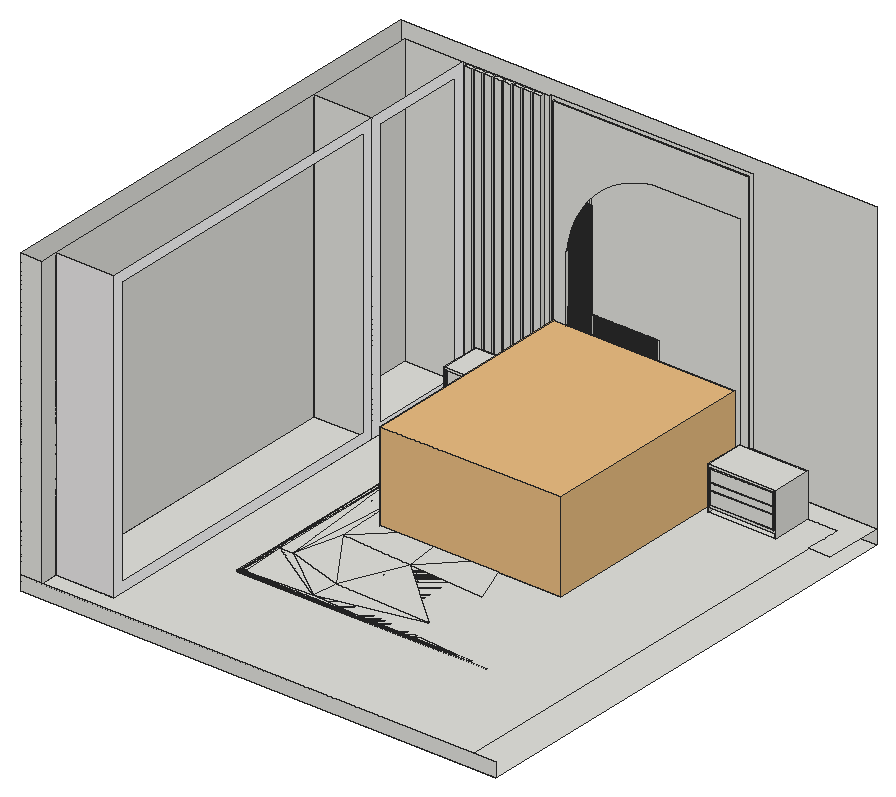
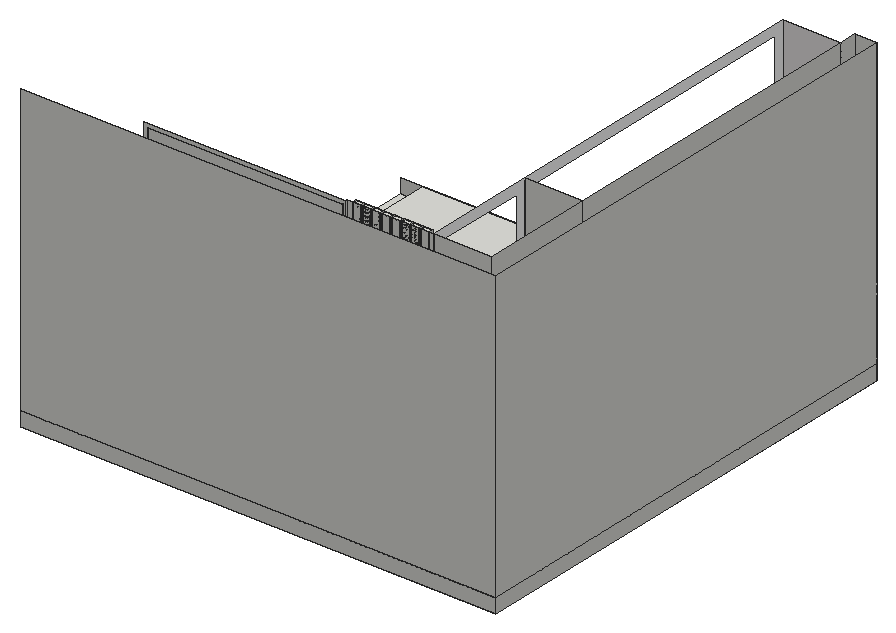
# SketchUp Ruby script. Lengths in inches.
U = 1.inch
M = Sketchup.active_model
def pt(a) = Geom::Point3d.new(a.map { |v| v * U })
def face(e, loops, mat)
  f = e.add_face(loops[0].map { |a| pt(a) })
  loops[1..].each { |l| e.add_face(l.map { |a| pt(a) }).erase! }
  f.material = f.back_material = mat if mat
  f
end
# faces: each face lists its corners as indices into pts; further lists are holes
def faces(e, pts, list, mat = nil) = list.each { |f| face(e, (f[0].is_a?(Array) ? f : [f]).map { |l| l.map { |i| pts[i] } }, mat) }
# xy, xz, yz: faces in a plane at the given z, y or x. An outline is a flat list of corners, or four numbers for a rectangle; further outlines are holes
def ring(l) = l.size == 4 ? [[l[0], l[1]], [l[2], l[1]], [l[2], l[3]], [l[0], l[3]]] : l.each_slice(2).to_a
def flat(e, list, mat, &to3) = list.each { |f| face(e, (f[0].is_a?(Array) ? f : [f]).map { |l| ring(l).map { |u, v| to3.(u, v) } }, mat) }
def xy(e, z, list, mat = nil) = flat(e, list, mat) { |x, y| [x, y, z] }
def xz(e, y, list, mat = nil) = flat(e, list, mat) { |x, z| [x, y, z] }
def yz(e, x, list, mat = nil) = flat(e, list, mat) { |y, z| [x, y, z] }
def lines(e, pts, list) = list.each { |a, b| e.add_line(pt(pts[a]), pt(pts[b])) }
# prism: a flat outline (further loops are holes) pulled along v
def prism(e, loops, v, mat = nil)
  f = face(e, loops, mat); d = Geom::Vector3d.new(v.map { |x| x * U })
  f.pushpull(f.normal.samedirection?(d) ? d.length : -d.length)
end
def box(e, o, s, mat = nil) = prism(e, [[o, [o[0] + s[0], o[1], o[2]], [o[0] + s[0], o[1] + s[1], o[2]], [o[0], o[1] + s[1], o[2]]]], [0, 0, s[2]], mat)
def at(x, y, z, deg = 0) = Geom::Transformation.translation(pt([x, y, z])) * Geom::Transformation.rotation(ORIGIN, Z_AXIS, deg.degrees)
def axes(o, x, y, z) = Geom::Transformation.new([*x, 0, *y, 0, *z, 0, *pt(o).to_a, 1])
def part(name) = M.definitions.add(name)
# library, detail: a bought-in or finely detailed component or shape, given as its bounding box
def library(name, o, s) = part(name).tap { |d| box(d.entities, o, s) }
def detail(e, o, s) = box(e.add_group.entities, o, s)
def put(e, d, t, mat = nil) = e.add_instance(d, t).tap { |i| i.material = mat if mat }
def group(e, t, mat = nil) = e.add_group.tap { |g| g.transformation = t; g.material = mat if mat }.entities
root = M.entities
M.materials.add("Generic").color = [234, 232, 232]
M.materials.add("[Color M00]").color = [255, 255, 255]
c1 = library("Bed 001",[-37.84,-46.07,0],[75.19,90.39,37.01])
xy(root,-6,[[0,0,198,198]])
xy(root,0,[[0,0,9,0,9,189,69.06,189,69.06,189.875,153.17,189.875,153.17,189,171.08,189,171.08,190.5,173.42,190.5,173.42,189,189,189,189,174,198,174,198,198,0,198],[9,0,189,0,189,189,176.63,189,176.63,172.375,148.19,172.375,148.19,189,153.17,189,153.17,189.875,69.06,189.875,69.06,189,33,189,33,7.36,9,7.36],[9,7.36,33,141.67],[54.68,45.79,53.76,45.82,54.37,46.18],[54.68,45.79,54.37,46.18,54.98,46.18],
  [54.68,45.79,54.98,46.18,71.8,46.18],[54.68,45.79,71.8,46.18,79.4375,45.79],[79.4375,45.79,71.8,46.18,129.55,46.18],[53.76,45.82,53.42,45.84,53.76,46.18],[53.76,45.82,53.76,46.18,54.37,46.18],
  [53.42,45.84,53.4,46.18,53.76,46.18],[53.4,46.18,53.37,47.09,53.76,46.79],[53.4,46.18,53.76,46.79,53.76,46.18],[53.76,46.18,53.76,46.79,54.37,46.18],[54.37,46.18,53.76,46.79,54.37,46.79],
  [54.37,46.18,54.37,46.79,54.98,46.18],[54.98,46.18,54.37,46.79,54.98,46.79],[54.98,46.18,54.98,46.79,70.45,46.79],[54.98,46.18,70.45,46.79,71.8,46.18],[71.8,46.18,70.45,46.79,142.125,46.79],
  [53.76,46.79,53.37,47.09,53.76,47.4],[53.76,46.79,53.76,47.4,54.37,46.79],[54.37,46.79,53.76,47.4,54.37,47.4],[54.37,46.79,54.37,47.4,54.98,46.79],[54.98,46.79,54.37,47.4,54.98,47.97],
  [54.98,46.79,54.98,47.97,68.23,47.4],[54.98,46.79,68.23,47.4,70.45,46.79],[70.45,46.79,68.23,47.4,143.14,47.4],[53.37,47.09,53.37,74.72,53.76,74.26],[53.37,47.09,53.76,74.26,53.76,47.4],
  [53.76,47.4,53.76,74.26,54.37,47.4],[54.37,47.4,53.76,74.26,54.37,100.67],[54.37,47.4,54.37,100.67,54.98,47.97],[68.23,47.4,54.98,47.97,75.08,53.77],[68.23,47.4,75.08,53.77,143.14,47.4],
  [54.98,47.97,54.37,100.67,54.98,109.7],[54.98,47.97,54.98,109.7,60.51,69.42],[54.98,47.97,60.51,69.42,75.08,53.77],[149.74,51.96,75.08,53.77,112.4,68.43],[75.08,53.77,60.51,69.42,92.35,73.72],
  [75.08,53.77,92.35,73.72,112.4,68.43],[112.4,68.43,80.56,101.52,111.5,116.5625],[112.4,68.43,92.35,73.72,80.56,101.52],[60.51,69.42,54.98,109.7,58.56,109.53],[60.51,69.42,58.56,109.53,80.56,101.52],
  [60.51,69.42,80.56,101.52,92.35,73.72],[53.76,74.26,53.37,74.72,53.76,118.57],[53.76,74.26,53.76,118.57,54.37,100.67],[53.37,74.72,53.37,122.82,53.76,118.57],[54.37,100.67,53.76,118.57,54.37,134.57],
  [54.37,100.67,54.37,134.57,54.98,109.7],[80.56,101.52,58.56,109.53,80.27,123.75],[80.56,101.52,80.27,123.75,111.5,116.5625],[58.56,109.53,54.98,109.7,67.21,132.46],[58.56,109.53,67.21,132.46,80.27,123.75],
  [54.98,109.7,54.37,134.57,54.98,134.57],[54.98,109.7,54.98,134.57,67.21,132.46],[111.5,116.5625,67.21,132.46,139.65,129.14],[111.5,116.5625,80.27,123.75,67.21,132.46],[53.76,118.57,53.37,122.82,53.76,134.57],
  [53.76,118.57,53.76,134.57,54.37,134.57],[53.37,122.82,53.37,134.87,53.76,134.57],[67.21,132.46,54.98,134.57,63.67,134.57],[67.21,132.46,63.67,134.57,139.03,134.57],[53.76,134.57,53.37,134.87,53.76,135.18],
  [53.76,134.57,53.76,135.18,54.37,134.57],[54.37,134.57,53.76,135.18,54.37,135.18],[54.37,134.57,54.37,135.18,54.98,134.57],[54.98,134.57,54.37,135.18,54.98,135.18],[54.98,134.57,54.98,135.18,63.67,134.57],
  [63.67,134.57,54.98,135.18,68.35,135.18],[63.67,134.57,68.35,135.18,139.03,134.57],[139.03,134.57,68.35,135.18,110.28,135.18],[53.37,134.87,53.4,135.79,53.76,135.18],[53.76,135.18,53.4,135.79,53.76,135.79],
  [53.76,135.18,53.76,135.79,54.37,135.18],[54.37,135.18,53.76,135.79,54.37,135.79],[54.37,135.18,54.37,135.79,54.98,135.18],[54.98,135.18,54.37,135.79,54.98,135.79],[54.98,135.18,54.98,135.79,63.62,135.79],
  [54.98,135.18,63.62,135.79,68.35,135.18],[68.35,135.18,63.62,135.79,92.94,135.79],[68.35,135.18,92.94,135.79,110.28,135.18],[53.4,135.79,53.76,136.14,53.76,135.79],[53.76,135.79,53.76,136.14,54.37,135.79],
  [54.37,135.79,53.76,136.14,54.68,136.17],[54.37,135.79,54.68,136.17,54.98,135.79],[54.98,135.79,54.68,136.17,63.62,135.79],[63.62,135.79,54.68,136.17,69.16,136.17],[63.62,135.79,69.16,136.17,92.94,135.79],
  [92.94,135.79,69.16,136.17,140.64,136.17],[9,141.67,33,189]])
xy(root,0.23,[[54.68,45.79,54.37,46.18,53.76,45.82],[54.68,45.79,54.98,46.18,54.37,46.18],[54.68,45.79,63.62,46.18,54.98,46.18],[54.68,45.79,78.85,45.79,63.62,46.18],[78.85,45.79,96.94,46.18,63.62,46.18],
  [78.85,45.79,157.71,45.79,96.94,46.18],[53.76,45.82,53.76,46.18,53.4,46.18],[53.76,45.82,54.37,46.18,53.76,46.18],[53.4,46.18,53.76,46.79,53.37,47.09],[53.4,46.18,53.76,46.18,53.76,46.79],
  [53.76,46.18,54.37,46.18,54.37,46.79],[53.76,46.18,54.37,46.79,53.76,46.79],[54.37,46.18,54.98,46.18,54.98,46.79],[54.37,46.18,54.98,46.79,54.37,46.79],[54.98,46.18,63.62,46.18,54.98,46.79],
  [63.62,46.18,75.59,46.79,54.98,46.79],[63.62,46.18,96.94,46.18,75.59,46.79],[96.94,46.18,150.44,46.79,75.59,46.79],[53.76,46.79,53.76,47.4,53.37,47.09],[53.76,46.79,54.37,46.79,54.37,47.4],
  [53.76,46.79,54.37,47.4,53.76,47.4],[54.37,46.79,54.98,46.79,54.37,47.4],[54.98,46.79,55.67,47.4,54.37,47.4],[54.98,46.79,75.59,46.79,55.67,47.4],[75.59,46.79,101.08,47.4,55.67,47.4],
  [75.59,46.79,150.44,46.79,101.08,47.4],[53.37,47.09,53.76,47.4,53.76,65.64],[53.37,47.09,53.76,65.64,53.37,73.96],[53.76,47.4,54.37,47.4,53.76,65.64],[54.37,47.4,54.37,73.58,53.76,65.64],
  [54.37,47.4,54.98,66.1,54.37,73.58],[54.37,47.4,55.67,47.4,54.98,66.1],[55.67,47.4,82.99,48.58,54.98,66.1],[55.67,47.4,101.08,47.4,82.99,48.58],[82.99,48.58,60.05,66.7,54.98,66.1],
  [82.99,48.58,84.18,59.15,60.05,66.7],[82.99,48.58,124,57.84,84.18,59.15],[124,57.84,94.82,84.31,84.18,59.15],[84.18,59.15,65.59,86,60.05,66.7],[84.18,59.15,94.82,84.31,65.59,86],
  [53.76,65.64,53.76,118.73,53.37,73.96],[53.76,65.64,54.37,73.58,53.76,118.73],[54.98,66.1,54.98,126.34,54.37,73.58],[54.98,66.1,60.05,66.7,54.98,126.34],[60.05,66.7,64.72,113.81,54.98,126.34],
  [60.05,66.7,65.59,86,64.72,113.81],[54.37,73.58,54.37,127.23,53.76,118.73],[54.37,73.58,54.98,126.34,54.37,127.23],[53.37,73.96,53.76,118.73,53.37,122.53],[126.68,81.95,117.31,106.81,94.82,84.31],
  [94.82,84.31,91.64,111.34,65.59,86],[94.82,84.31,117.31,106.81,91.64,111.34],[65.59,86,91.64,111.34,64.72,113.81],[117.31,106.81,111.91,130.52,91.64,111.34],[91.64,111.34,66.5,131.22,64.72,113.81],
  [91.64,111.34,111.91,130.52,66.5,131.22],[64.72,113.81,66.5,131.22,54.98,126.34],[53.76,118.73,53.76,134.57,53.37,122.53],[53.76,118.73,54.37,127.23,53.76,134.57],[53.37,122.53,53.76,134.57,53.37,134.87],
  [54.98,126.34,54.98,134.57,54.37,127.23],[54.98,126.34,60.14,134.57,54.98,134.57],[54.98,126.34,66.5,131.22,60.14,134.57],[54.37,127.23,54.37,134.57,53.76,134.57],[54.37,127.23,54.98,134.57,54.37,134.57],
  [111.91,130.52,92.98,134.57,66.5,131.22],[66.5,131.22,92.98,134.57,60.14,134.57],[53.76,134.57,53.76,135.18,53.37,134.87],[53.76,134.57,54.37,134.57,54.37,135.18],[53.76,134.57,54.37,135.18,53.76,135.18],
  [54.37,134.57,54.98,134.57,54.98,135.18],[54.37,134.57,54.98,135.18,54.37,135.18],[54.98,134.57,60.14,134.57,54.98,135.18],[60.14,134.57,68.15,135.18,54.98,135.18],[60.14,134.57,92.98,134.57,68.15,135.18],
  [92.98,134.57,121.1,135.18,68.15,135.18],[53.37,134.87,53.76,135.18,53.4,135.79],[53.76,135.18,53.76,135.79,53.4,135.79],[53.76,135.18,54.37,135.18,54.37,135.79],[53.76,135.18,54.37,135.79,53.76,135.79],
  [54.37,135.18,54.98,135.18,54.98,135.79],[54.37,135.18,54.98,135.79,54.37,135.79],[54.98,135.18,63.62,135.79,54.98,135.79],[54.98,135.18,68.15,135.18,63.62,135.79],[68.15,135.18,89.4,135.79,63.62,135.79],
  [68.15,135.18,121.1,135.18,89.4,135.79],[53.4,135.79,53.76,135.79,53.42,136.125],[53.76,135.79,53.76,136.14,53.42,136.125],[53.76,135.79,54.37,135.79,53.76,136.14],[54.37,135.79,54.68,136.17,53.76,136.14],
  [54.37,135.79,54.98,135.79,54.68,136.17],[54.98,135.79,63.62,135.79,54.68,136.17],[63.62,135.79,67.51,136.17,54.68,136.17],[63.62,135.79,89.4,135.79,67.51,136.17],[89.4,135.79,115.29,136.17,67.51,136.17],
  [89.4,135.79,134.45,135.79,115.29,136.17]])
xy(root,1.3,[[70.35,189,76.0625,189.875],[76.0625,189.8125,76.6,189.875],[77,189.8125,77.6,189.875],[78,189.8125,78.6,189.875],[79,189.8125,79.6,189.875],
  [80,189.8125,80.6,189.875],[81,189.8125,81.6,189.875],[82.17,189.8125,82.77,189.875],[83.33,189.8125,83.93,189.875],[84.49,189.8125,85.09,189.875],
  [85.66,189.8125,86.26,189.875],[86.82,189.8125,87.42,189.875],[87.99,189.8125,88.58,189.875],[89.15,189.8125,89.75,189.875],[90.3125,189.8125,90.91,189.875],
  [91.48,189.8125,92.08,189.875],[92.64,189.8125,93.24,189.875],[93.8,189.8125,94.4,189.875],[94.97,189.8125,95.57,189.875],[96.13,189.8125,96.73,189.875],
  [97.29,189.8125,97.89,189.875],[98.46,189.8125,99.06,189.875],[99.62,189.8125,100.22,189.875],[100.79,189.8125,101.38,189.875],[101.95,189.8125,102.55,189.875],
  [103.11,189.8125,103.71,189.875],[104.28,189.8125,104.875,189.875],[105.28,189.8125,105.875,189.875],[106.28,189.8125,106.875,189.875],[107.28,189.8125,107.875,189.875],
  [108.28,189.8125,108.875,189.875],[109.28,189.8125,109.875,189.875],[110.28,189.8125,110.875,189.875],[111.28,189.8125,111.875,189.875],[112.28,189.8125,112.875,189.875],
  [113.28,189.8125,113.875,189.875]])
xz(root,0,[[0,-6,198,0],[0,0,9,120]])
xz(root,7.36,[[9,0,33,120]],"Generic")
xz(root,45.79,[[54.68,0,78.85,0.23,54.68,0.23],[54.68,0,79.4375,0,78.85,0.23],[79.4375,0,156.43,0,78.85,0.23]])
xz(root,136.17,[[54.68,0,54.68,0.23,67.51,0.23],[54.68,0,67.51,0.23,69.16,0],[69.16,0,67.51,0.23,115.29,0.23],[69.16,0,115.29,0.23,140.64,0]])
xz(root,141.67,[[9,0,33,120]])
xz(root,189,[[9,0,33,120],[33,0,35.02,120],[38.39,0,69.06,120],[70.35,1.3,76.0625,1.3,76.0625,64.2,76.79,68.84,78.03,73.375,79.76,77.74,81.96,81.89,84.62,85.77,87.68,89.33,91.12,92.53,94.89,95.33,98.95,97.7,103.25,99.6,107.73,101.01,112.34,101.92,148.625,101.92,148.625,1.3,151.87,1.3,151.87,118.7,70.35,118.7]])
xz(root,189.8125,[[76.0625,1.3,76.6,1.3,76.6,67.64,76.0625,64.2],[77,1.3,77.6,1.3,77.6,71.82,77,69.625],[78,1.3,78.6,1.3,78.6,74.82,78.03,73.375,78,73.29],[79,1.3,79.6,1.3,79.6,77.35,79,75.84],[80,1.3,80.6,1.3,80.6,79.33,80,78.2],
  [81,1.3,81.6,1.3,81.6,81.21,81,80.08],[82.17,1.3,82.77,1.3,82.77,83.06,82.17,82.1875],[83.33,1.3,83.93,1.3,83.93,84.67,83.86,84.67,83.33,83.89],[84.49,1.3,85.09,1.3,85.09,84.67,84.875,84.67,84.875,86.07,84.62,85.77,84.28,85.28,84.28,84.67,84.49,84.67],[85.66,1.3,86.26,1.3,86.26,44.04,86.13,44.04,86.13,84.67,85.875,84.67,85.875,87.24,85.28,86.54,85.28,84.67,85.66,84.67],
  [86.82,1.3,87.42,44.04],[87.99,1.3,88.58,44.04],[89.15,1.3,89.75,44.04],[90.3125,1.3,90.91,44.04],[91.48,1.3,92.08,44.04],
  [92.64,1.3,93.24,44.04],[93.8,1.3,94.4,44.04],[94.97,1.3,95.57,44.04],[96.13,1.3,96.73,44.04],[97.29,1.3,97.89,44.04],
  [98.46,1.3,99.06,44.04],[99.62,1.3,100.22,44.04],[100.79,1.3,101.38,44.04],[101.95,1.3,102.55,44.04],[103.11,1.3,103.71,44.04],
  [104.28,1.3,104.875,44.04],[105.28,1.3,105.875,44.04],[106.28,1.3,106.875,44.04],[107.28,1.3,107.875,44.04],[108.28,1.3,108.875,44.04],
  [109.28,1.3,109.875,44.04],[110.28,1.3,110.875,44.04],[111.28,1.3,111.875,44.04],[112.28,1.3,112.875,44.04],[113.28,1.3,113.875,44.04]])
xz(root,189.875,[[[69.06,0,153.17,120],[70.35,1.3,151.87,118.7]],[71,1.3,71.6,44.04],[72,1.3,72.6,44.04],[73,1.3,73.6,44.04],[74,1.3,74.6,44.04],
  [75,1.3,75.6,44.04],[76,1.3,76.0625,44.04],[76.6,1.3,77,1.3,77,69.625,76.79,68.84,76.6,67.64],[77.6,1.3,78,1.3,78,73.29,77.6,71.82],[78.6,1.3,79,1.3,79,75.84,78.6,74.82],
  [79.6,1.3,80,1.3,80,78.2,79.76,77.74,79.6,77.35],[80.6,1.3,81,1.3,81,80.08,80.6,79.33],[81.6,1.3,82.17,1.3,82.17,82.1875,81.96,81.89,81.6,81.21],[82.77,1.3,83.33,1.3,83.33,83.89,82.77,83.06],[83.93,1.3,84.49,1.3,84.49,84.67,84.28,84.67,84.28,85.28,83.86,84.67,83.93,84.67],
  [85.09,1.3,85.66,1.3,85.66,84.67,85.28,84.67,85.28,86.54,84.875,86.07,84.875,84.67,85.09,84.67],[86.26,1.3,86.82,44.04],[87.42,1.3,87.99,44.04],[88.58,1.3,89.15,44.04],[89.75,1.3,90.3125,44.04],
  [90.91,1.3,91.48,44.04],[92.08,1.3,92.64,44.04],[93.24,1.3,93.8,44.04],[94.4,1.3,94.97,44.04],[95.57,1.3,96.13,44.04],
  [96.73,1.3,97.29,44.04],[97.89,1.3,98.46,44.04],[99.06,1.3,99.62,44.04],[100.22,1.3,100.79,44.04],[101.38,1.3,101.95,44.04],
  [102.55,1.3,103.11,44.04],[103.71,1.3,104.28,44.04],[104.875,1.3,105.28,44.04],[105.875,1.3,106.28,44.04],[106.875,1.3,107.28,44.04],
  [107.875,1.3,108.28,44.04],[108.875,1.3,109.28,44.04],[109.875,1.3,110.28,44.04],[110.875,1.3,111.28,44.04],[111.875,1.3,112.28,44.04],
  [112.875,1.3,113.28,44.04]])
xz(root,198,[[0,-6,198,0],[0,0,198,120]])
yz(root,0,[[0,-6,198,0],[0,0,198,120]])
yz(root,9,[[0,0,7.36,120],[7.36,0,141.67,120],[141.67,0,189,120]])
yz(root,33,[[[7.36,0,141.67,120],[11.43,4.07,137.59,115.93]],[[141.67,0,189,120],[145.84,4.17,184.83,115.83]]],"[Color M00]")
yz(root,53.37,[[47.09,0,47.09,0.23,73.96,0.23],[47.09,0,73.96,0.23,74.72,0],[74.72,0,73.96,0.23,122.53,0.23],[74.72,0,122.53,0.23,122.82,0],[122.82,0,122.53,0.23,134.87,0.23],
  [122.82,0,134.87,0.23,134.87,0]])
yz(root,69.06,[[189,0,189.875,120]])
yz(root,70.35,[[189,1.3,189.875,118.7]])
yz(root,76.0625,[[189,1.3,189.8125,64.2],[189.8125,1.3,189.875,44.04]])
yz(root,76.6,[[189.8125,1.3,189.875,67.64]])
yz(root,77,[[189.8125,1.3,189.875,69.625]])
yz(root,77.6,[[189.8125,1.3,189.875,71.82]])
yz(root,78,[[189.8125,1.3,189.875,73.29]])
yz(root,78.6,[[189.8125,1.3,189.875,74.82]])
yz(root,79,[[189.8125,1.3,189.875,75.84]])
yz(root,79.6,[[189.8125,1.3,189.875,77.35]])
yz(root,80,[[189.8125,1.3,189.875,78.2]])
yz(root,80.6,[[189.8125,1.3,189.875,79.33]])
yz(root,81,[[189.8125,1.3,189.875,80.08]])
yz(root,81.6,[[189.8125,1.3,189.875,81.21]])
yz(root,82.17,[[189.8125,1.3,189.875,82.1875]])
yz(root,82.77,[[189.8125,1.3,189.875,83.06]])
yz(root,83.33,[[189.8125,1.3,189.875,83.89]])
yz(root,83.93,[[189.8125,1.3,189.875,84.67]])
yz(root,84.49,[[189.8125,1.3,189.875,84.67]])
yz(root,85.09,[[189.8125,1.3,189.875,84.67]])
yz(root,85.66,[[189.8125,1.3,189.875,84.67]])
yz(root,86.26,[[189.8125,1.3,189.875,44.04]])
yz(root,86.82,[[189.8125,1.3,189.875,44.04]])
yz(root,87.42,[[189.8125,1.3,189.875,44.04]])
yz(root,87.99,[[189.8125,1.3,189.875,44.04]])
yz(root,88.58,[[189.8125,1.3,189.875,44.04]])
yz(root,89.15,[[189.8125,1.3,189.875,44.04]])
yz(root,89.75,[[189.8125,1.3,189.875,44.04]])
yz(root,90.3125,[[189.8125,1.3,189.875,44.04]])
yz(root,90.91,[[189.8125,1.3,189.875,44.04]])
yz(root,91.48,[[189.8125,1.3,189.875,44.04]])
yz(root,92.08,[[189.8125,1.3,189.875,44.04]])
yz(root,92.64,[[189.8125,1.3,189.875,44.04]])
yz(root,93.24,[[189.8125,1.3,189.875,44.04]])
yz(root,93.8,[[189.8125,1.3,189.875,44.04]])
yz(root,94.4,[[189.8125,1.3,189.875,44.04]])
yz(root,94.97,[[189.8125,1.3,189.875,44.04]])
yz(root,95.57,[[189.8125,1.3,189.875,44.04]])
yz(root,96.13,[[189.8125,1.3,189.875,44.04]])
yz(root,96.73,[[189.8125,1.3,189.875,44.04]])
yz(root,97.29,[[189.8125,1.3,189.875,44.04]])
yz(root,97.89,[[189.8125,1.3,189.875,44.04]])
yz(root,98.46,[[189.8125,1.3,189.875,44.04]])
yz(root,99.06,[[189.8125,1.3,189.875,44.04]])
yz(root,99.62,[[189.8125,1.3,189.875,44.04]])
yz(root,100.22,[[189.8125,1.3,189.875,44.04]])
yz(root,100.79,[[189.8125,1.3,189.875,44.04]])
yz(root,101.38,[[189.8125,1.3,189.875,44.04]])
yz(root,101.95,[[189.8125,1.3,189.875,44.04]])
yz(root,102.55,[[189.8125,1.3,189.875,44.04]])
yz(root,103.11,[[189.8125,1.3,189.875,44.04]])
yz(root,103.71,[[189.8125,1.3,189.875,44.04]])
yz(root,104.28,[[189.8125,1.3,189.875,44.04]])
yz(root,104.875,[[189.8125,1.3,189.875,44.04]])
yz(root,105.28,[[189.8125,1.3,189.875,44.04]])
yz(root,105.875,[[189.8125,1.3,189.875,44.04]])
yz(root,106.28,[[189.8125,1.3,189.875,44.04]])
yz(root,106.875,[[189.8125,1.3,189.875,44.04]])
yz(root,107.28,[[189.8125,1.3,189.875,44.04]])
yz(root,107.875,[[189.8125,1.3,189.875,44.04]])
yz(root,108.28,[[189.8125,1.3,189.875,44.04]])
yz(root,108.875,[[189.8125,1.3,189.875,44.04]])
yz(root,109.28,[[189.8125,1.3,189.875,44.04]])
yz(root,109.875,[[189.8125,1.3,189.875,44.04]])
yz(root,110.28,[[189.8125,1.3,189.875,44.04]])
yz(root,110.875,[[189.8125,1.3,189.875,44.04]])
yz(root,111.28,[[189.8125,1.3,189.875,44.04]])
yz(root,111.875,[[189.8125,1.3,189.875,44.04]])
yz(root,112.28,[[189.8125,1.3,189.875,44.04]])
yz(root,112.875,[[189.8125,1.3,189.875,44.04]])
yz(root,113.28,[[189.8125,1.3,189.875,44.04]])
p = [[53.4,46.18,0.23],[53.4,46.18,0],[53.42,45.84,0],[53.76,45.82,0.23],[53.76,45.82,0],[54.68,45.79,0.23],
  [54.68,45.79,0],[53.37,47.09,0.23],[53.37,47.09,0],[53.4,135.79,0],[53.37,134.87,0],[53.37,134.87,0.23],
  [53.4,135.79,0.23],[53.42,136.125,0.23],[53.76,136.14,0],[53.76,136.14,0.23],[54.68,136.17,0],[54.68,136.17,0.23]]
faces(root,p,[[0,1,2],[0,2,3],[2,4,3],[5,3,4],[4,6,5],[0,7,8],[8,1,0],[9,10,11],
  [11,12,9],[13,9,12],[9,13,14],[15,14,13],[16,14,15],[15,17,16]])
g1 = group(root,at(35.02,189,0))
box(g1,[0,-1.8125,0],[3.37,1.8125,120])
box(g1,[4.0625,-1.8125,0],[3.37,1.8125,120])
box(g1,[8.125,-1.8125,0],[3.375,1.8125,120])
box(g1,[12.1875,-1.8125,0],[3.37,1.8125,120])
box(g1,[16.25,-1.8125,0],[3.37,1.8125,120])
box(g1,[20.3125,-1.8125,0],[3.37,1.8125,120])
box(g1,[24.375,-1.8125,0],[3.375,1.8125,120])
box(g1,[28.4375,-1.8125,0],[3.37,1.8125,120])
put(root,c1,at(108.78,144.68,0))
g2 = group(root,at(148.19,172.375,0))
xy(g2,0,[[-107.125,-3.25,-107.125,13.375,-78.6875,13.375,-78.6875,-3.25,-79.125,-3.25,-79.125,4.625,-106.5,4.625,-106.5,-3.25],[0,0,0,16.625,28.4375,16.625,28.4375,0,28,0,28,7.875,0.625,7.875,0.625,0]])
xy(g2,1.84,[[-106.5,-3.25,-79.125,4.625],[0.625,0,28,7.875]])
xy(g2,2.62,[[-106.35,-3.25,-79.46,-2.5],[0.78,0,27.66,0.75]])
xy(g2,3.02,[[-105.95,-3.25,-79.86,-2.5],[1.18,0,27.26,0.75]])
xy(g2,8.23,[[-105.95,-3.25,-79.86,-2.5],[1.18,0,27.26,0.75]])
xy(g2,8.67,[[-105.95,-3.25,-79.86,-2.5],[1.18,0,27.26,0.75]])
xy(g2,11.21,[[-105.95,-3.25,-79.86,-2.5],[1.18,0,27.26,0.75]])
xy(g2,11.64,[[-105.95,-3.25,-79.86,-2.5],[1.18,0,27.26,0.75]])
xy(g2,16.54,[[-105.95,-3.25,-79.86,-2.5],[1.18,0,27.26,0.75]])
xy(g2,16.94,[[-106.35,-3.25,-79.46,-2.5],[0.78,0,27.66,0.75]])
xy(g2,17.72,[[-107.125,-3.25,-78.6875,13.375],[0,0,28.4375,16.625]])
xz(g2,-3.25,[[-107.125,0,-106.5,1.84],[-79.125,0,-78.6875,1.84],[[-107.125,1.84,-78.6875,17.72],[-106.35,2.62,-79.46,16.94]],[-105.95,3.02,-79.86,8.23],[-105.95,8.67,-79.86,11.21],
  [-105.95,11.64,-79.86,16.54]])
xz(g2,-2.5,[[[-106.35,2.62,-79.46,16.94],[-105.95,3.02,-79.86,16.54]],[-105.95,8.23,-79.86,8.67],[-105.95,11.21,-79.86,11.64]])
xz(g2,0,[[0,0,0.625,1.84],[28,0,28.4375,1.84],[[0,1.84,28.4375,17.72],[0.78,2.62,27.66,16.94]],[1.18,3.02,27.26,8.23],[1.18,8.67,27.26,11.21],
  [1.18,11.64,27.26,16.54]])
xz(g2,0.75,[[[0.78,2.62,27.66,16.94],[1.18,3.02,27.26,16.54]],[1.18,8.23,27.26,8.67],[1.18,11.21,27.26,11.64]])
xz(g2,4.625,[[-106.5,0,-79.125,1.84]])
xz(g2,7.875,[[0.625,0,28,1.84]])
xz(g2,13.375,[[-107.125,0,-102.15,17.72],[-102.15,0,-84.23,17.72],[-84.23,0,-81.89,17.72],[-81.89,0,-78.6875,17.72]])
xz(g2,16.625,[[0,0,4.98,17.72],[4.98,0,22.89,17.72],[22.89,0,25.23,17.72],[25.23,0,28.4375,17.72]])
yz(g2,-107.125,[[-3.25,0,13.375,17.72]])
yz(g2,-106.5,[[-3.25,0,4.625,1.84]])
yz(g2,-106.35,[[-3.25,2.62,-2.5,16.94]])
yz(g2,-105.95,[[-3.25,3.02,-2.5,8.23],[-3.25,8.67,-2.5,11.21],[-3.25,11.64,-2.5,16.54]])
yz(g2,-79.86,[[-3.25,3.02,-2.5,8.23],[-3.25,8.67,-2.5,11.21],[-3.25,11.64,-2.5,16.54]])
yz(g2,-79.46,[[-3.25,2.62,-2.5,16.94]])
yz(g2,-79.125,[[-3.25,0,4.625,1.84]])
yz(g2,-78.6875,[[-3.25,0,13.375,17.72]])
yz(g2,0,[[0,0,16.625,17.72]])
yz(g2,0.625,[[0,0,7.875,1.84]])
yz(g2,0.78,[[0,2.62,0.75,16.94]])
yz(g2,1.18,[[0,3.02,0.75,8.23],[0,8.67,0.75,11.21],[0,11.64,0.75,16.54]])
yz(g2,27.26,[[0,3.02,0.75,8.23],[0,8.67,0.75,11.21],[0,11.64,0.75,16.54]])
yz(g2,27.66,[[0,2.62,0.75,16.94]])
yz(g2,28,[[0,0,7.875,1.84]])
yz(g2,28.4375,[[0,0,16.625,17.72]])
